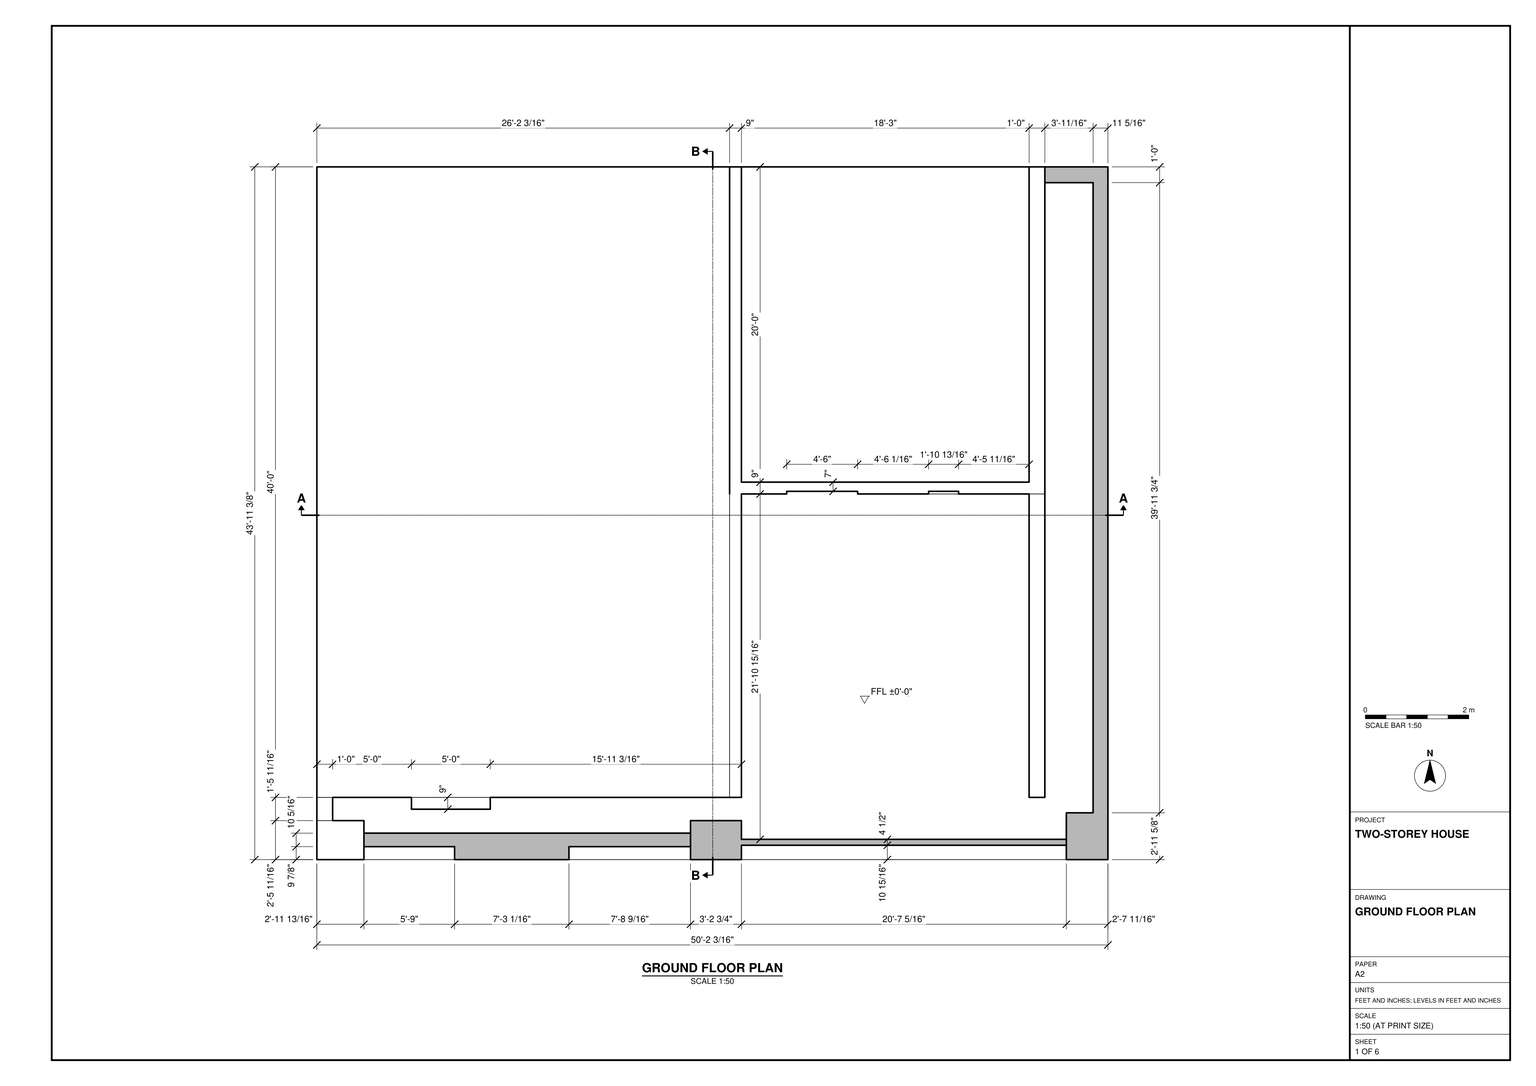
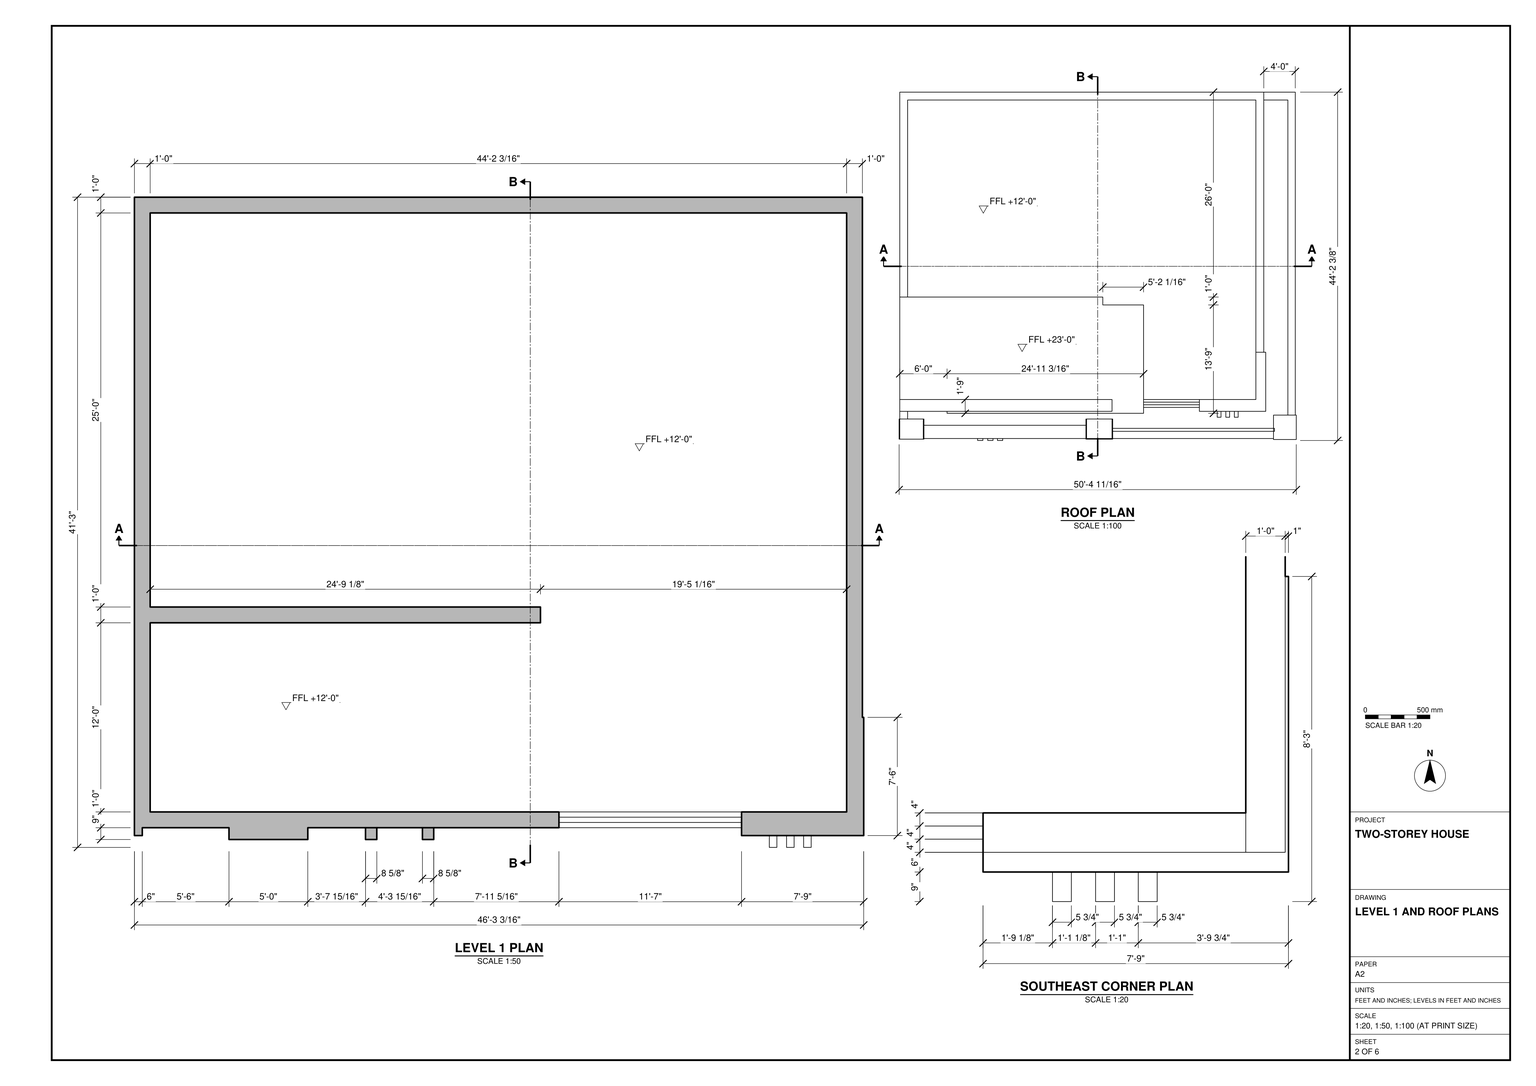
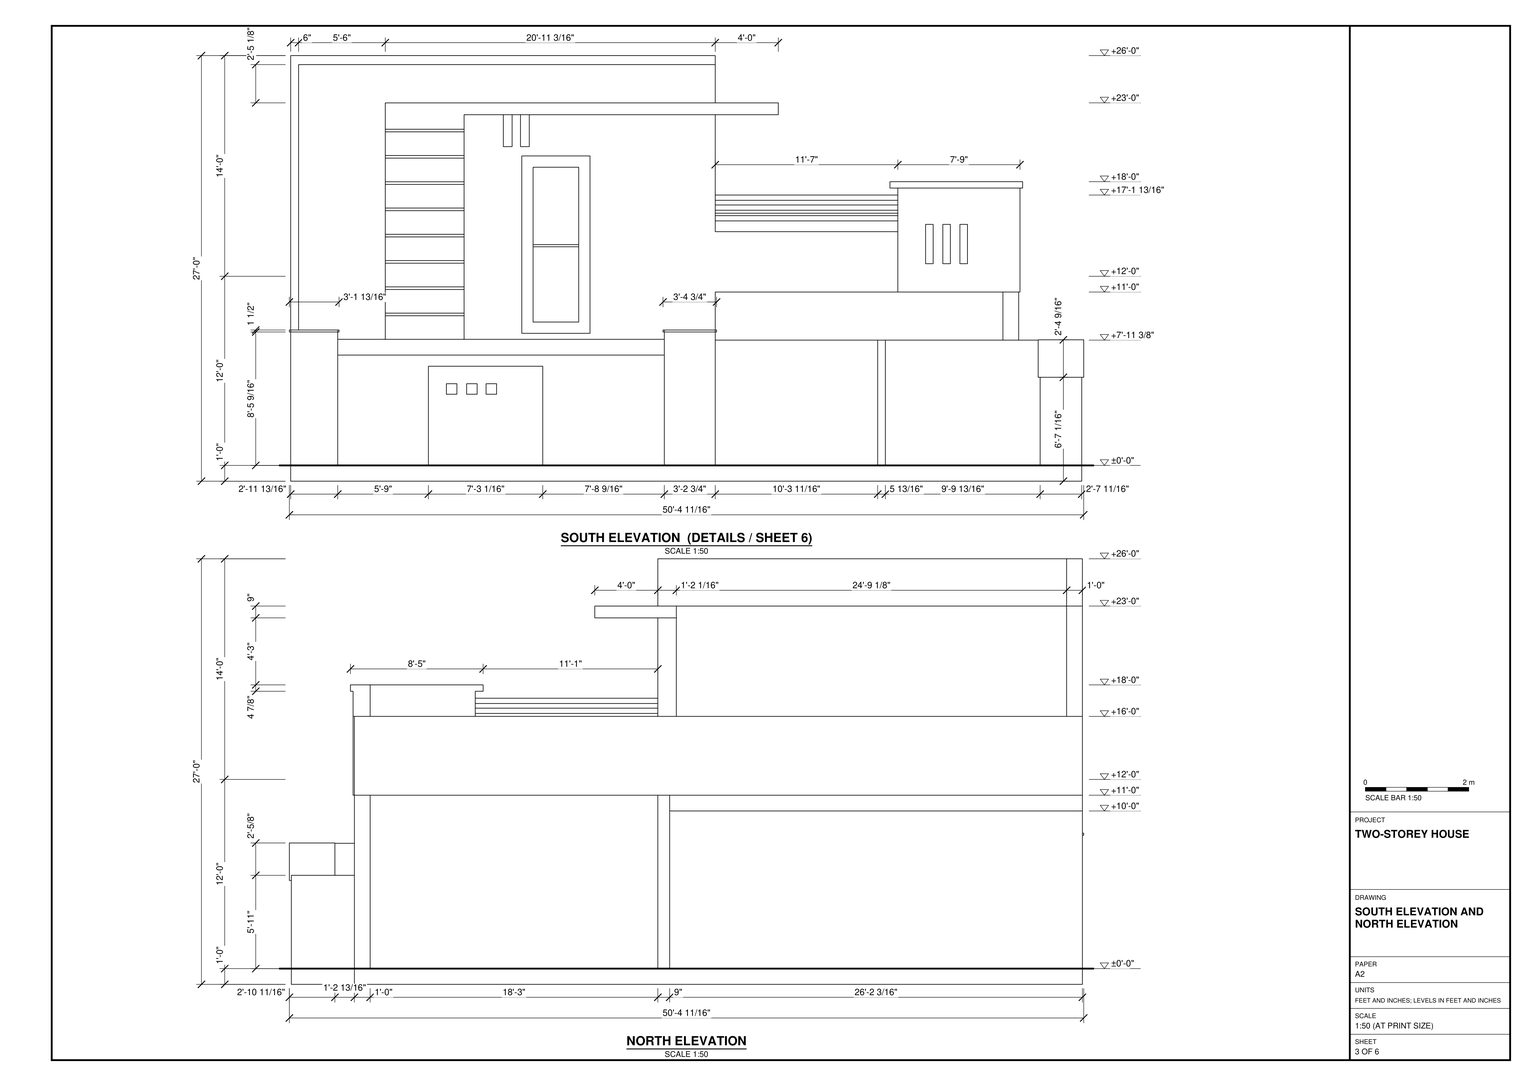
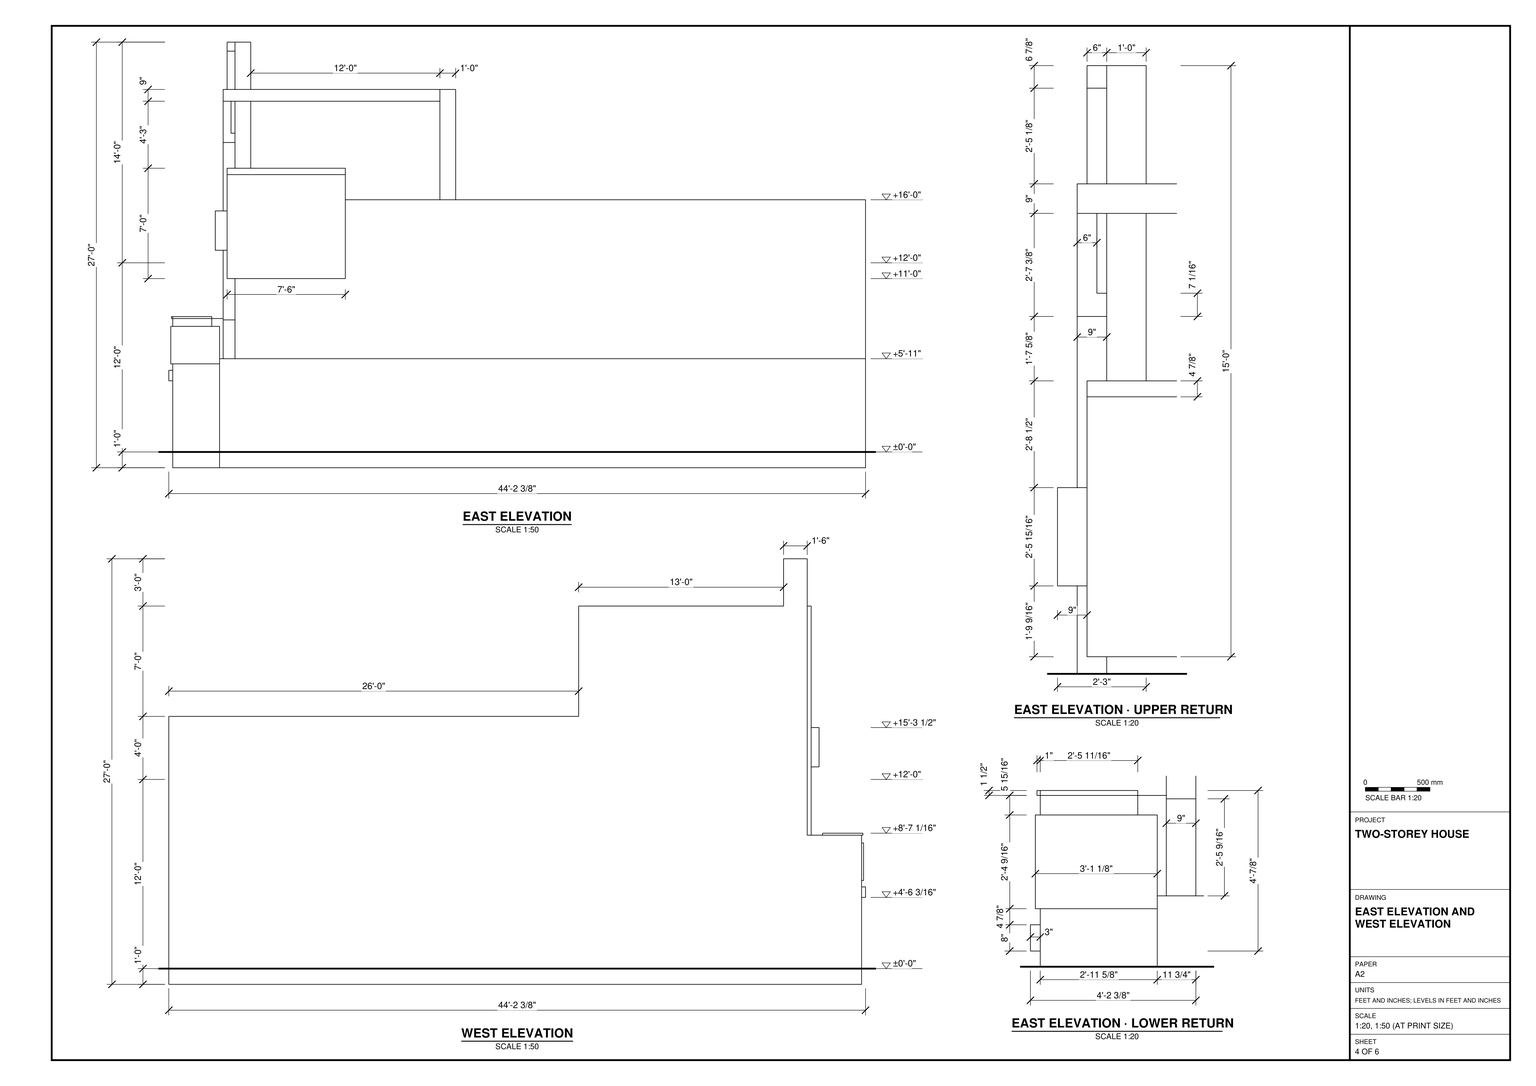
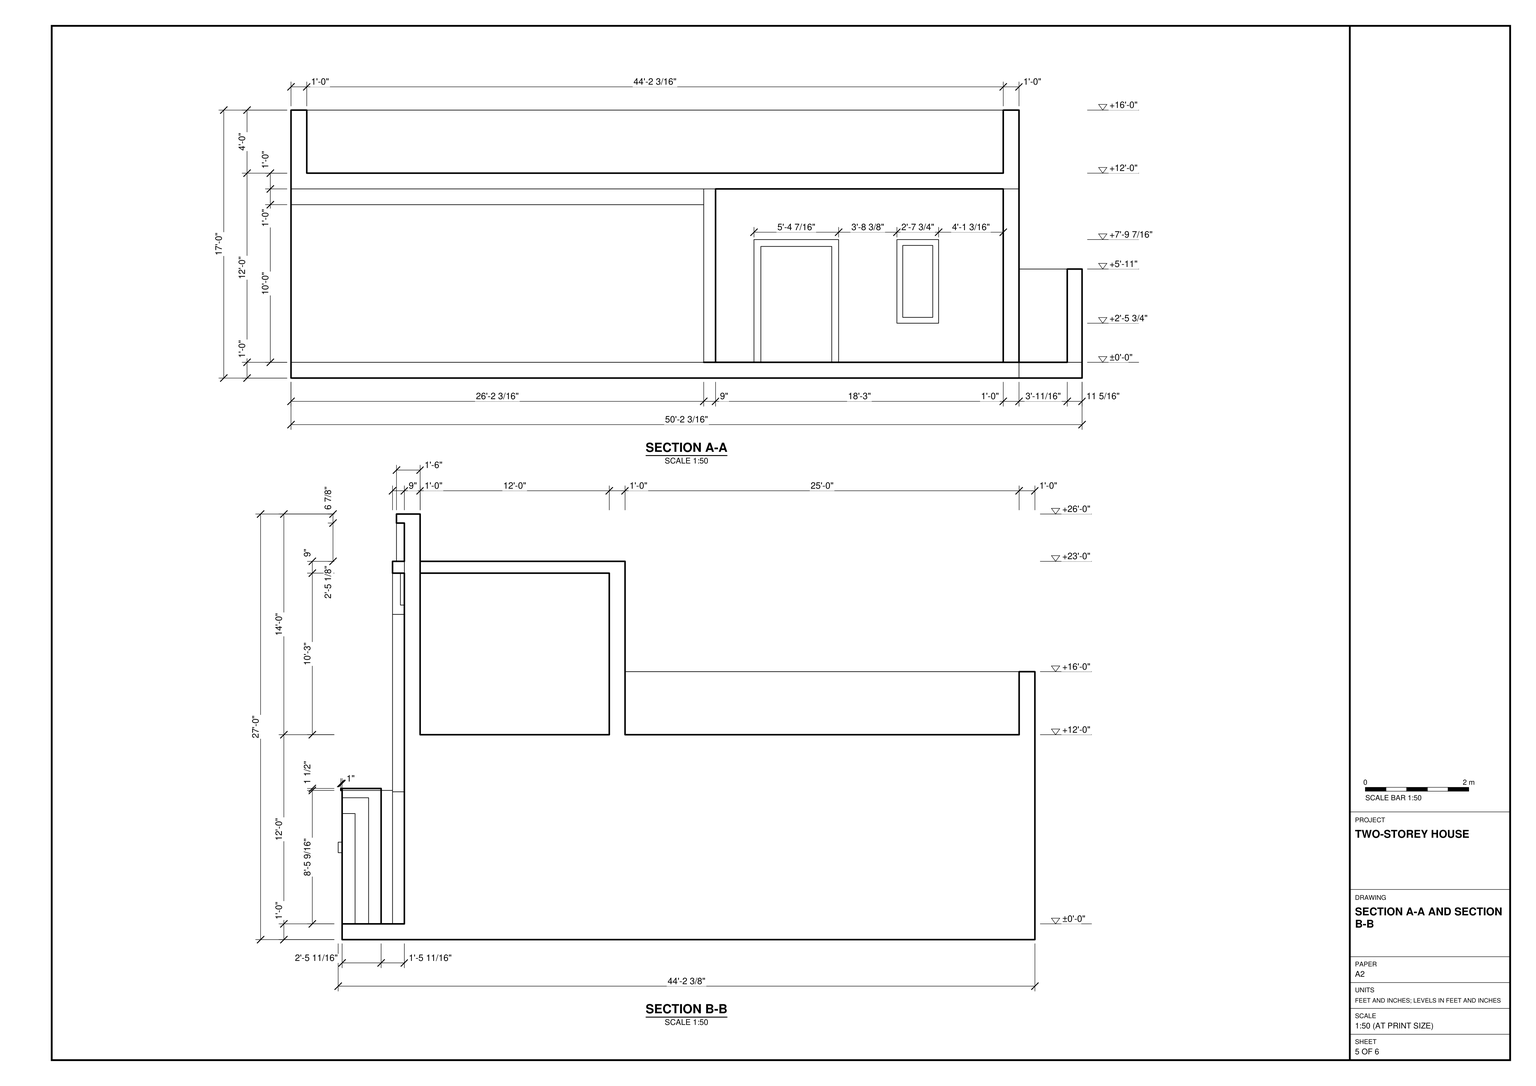
Use task_files/diagram_01.pdf to model the two-storey house in SketchUp. Work in feet and inches. The overall model must measure 50'-4 11/16" east to west, 44'-2 3/8" north to south and 27'-0" from the underside of the base to the highest point. Set the ground-floor finished level at ±0'-0" and the upper floor at +12'-0".

Lay out the broad west bay and the narrower east bay, including the cross wall that divides the east bay. Follow the plans for wall thicknesses, slab edges and openings. Use the roof plan and elevations together to locate the taller front volume, its projecting flat roof and the lower terrace. On the south face, model the horizontal bands beside the tall framed opening. Continue the terrace railing to the solid southeast corner and use the enlarged corner plan to place its narrow vertical details. Model the front boundary wall, piers and gate separately from the house facade, retaining the setbacks shown in plan.

Keep shell elements such as walls, slabs and roof pieces in separate groups or components. Keep each furniture or joinery piece shown separate and use components for repeated parts. Any decor or loose items shown may use suitable library components. Save one SketchUp model as output_files/two_storey_house_with_a_stepped_flat_roof.skp.

# SketchUp Ruby script. Lengths in inches.
U = 1.inch
M = Sketchup.active_model
def pt(a) = Geom::Point3d.new(a.map { |v| v * U })
def face(e, loops, mat)
  f = e.add_face(loops[0].map { |a| pt(a) })
  loops[1..].each { |l| e.add_face(l.map { |a| pt(a) }).erase! }
  f.material = f.back_material = mat if mat
  f
end
# faces: each face lists its corners as indices into pts; further lists are holes
def faces(e, pts, list, mat = nil) = list.each { |f| face(e, (f[0].is_a?(Array) ? f : [f]).map { |l| l.map { |i| pts[i] } }, mat) }
# xy, xz, yz: faces in a plane at the given z, y or x. An outline is a flat list of corners, or four numbers for a rectangle; further outlines are holes
def ring(l) = l.size == 4 ? [[l[0], l[1]], [l[2], l[1]], [l[2], l[3]], [l[0], l[3]]] : l.each_slice(2).to_a
def flat(e, list, mat, &to3) = list.each { |f| face(e, (f[0].is_a?(Array) ? f : [f]).map { |l| ring(l).map { |u, v| to3.(u, v) } }, mat) }
def xy(e, z, list, mat = nil) = flat(e, list, mat) { |x, y| [x, y, z] }
def xz(e, y, list, mat = nil) = flat(e, list, mat) { |x, z| [x, y, z] }
def yz(e, x, list, mat = nil) = flat(e, list, mat) { |y, z| [x, y, z] }
def lines(e, pts, list) = list.each { |a, b| e.add_line(pt(pts[a]), pt(pts[b])) }
# prism: a flat outline (further loops are holes) pulled along v
def prism(e, loops, v, mat = nil)
  f = face(e, loops, mat); d = Geom::Vector3d.new(v.map { |x| x * U })
  f.pushpull(f.normal.samedirection?(d) ? d.length : -d.length)
end
def box(e, o, s, mat = nil) = prism(e, [[o, [o[0] + s[0], o[1], o[2]], [o[0] + s[0], o[1] + s[1], o[2]], [o[0], o[1] + s[1], o[2]]]], [0, 0, s[2]], mat)
def at(x, y, z, deg = 0) = Geom::Transformation.translation(pt([x, y, z])) * Geom::Transformation.rotation(ORIGIN, Z_AXIS, deg.degrees)
def axes(o, x, y, z) = Geom::Transformation.new([*x, 0, *y, 0, *z, 0, *pt(o).to_a, 1])
def part(name) = M.definitions.add(name)
# library, detail: a bought-in or finely detailed component or shape, given as its bounding box
def library(name, o, s) = part(name).tap { |d| box(d.entities, o, s) }
def detail(e, o, s) = box(e.add_group.entities, o, s)
def put(e, d, t, mat = nil) = e.add_instance(d, t).tap { |i| i.material = mat if mat }
def group(e, t, mat = nil) = e.add_group.tap { |g| g.transformation = t; g.material = mat if mat }.entities
root = M.entities
M.materials.add("[0005_LightPink]").color = [255, 182, 193]
M.materials.add("[0008_LavenderBlush]").color = [204, 192, 195]
M.materials.add("[0012_Bisque]").color = [221, 198, 170]
M.materials.add("[0012_Bisque]1").color = [255, 228, 196]
M.materials.add("[0029_BlanchedAlmond]").color = [198, 183, 159]
M.materials.add("[0042_Sienna]").color = [56, 28, 15]
M.materials.add("[0111_SlateGray]").color = [112, 128, 144]
M.materials.add("[0132_LightGray]").color = [169, 169, 169]
M.materials.add("[0134_DimGray]").color = [105, 105, 105]
M.materials.add("[0136_Charcoal]").color = [35, 35, 35]
M.materials.add("[0137_Black]").color = [0, 0, 0]
M.materials.add("[Cladding Siding Tan]").color = [162, 126, 95]
M.materials.add("[Concrete Aggregate Smoke]").color = [154, 150, 148]
M.materials.add("[Stone Flagstone Ashlar]").color = [175, 116, 102]
M.materials.add("[Stone Marble]").color = [143, 138, 136]
M.materials.add("[Translucent Glass Blue]").color = [63, 94, 150]
M.materials["[Translucent Glass Blue]"].alpha = 0.5
M.materials.add("[Translucent Glass Gray]").color = [128, 128, 128]
M.materials["[Translucent Glass Gray]"].alpha = 0.5
xy(root,0,[[1,3,555.1875,50.375],[555.1875,3,603.1875,50.375],[1,50.375,555.1875,530.375],[555.1875,50.375,603.1875,530.375]])
xy(root,12,[[36.8125,3,105.84,12.87],[192.9,3,285.4375,12.87],[285.4375,3,285.4375,32.6875,324.1875,32.6875,324.1875,18.4375,571.53,18.4375,571.53,13.9375,324.1875,13.9375,324.1875,3],[73,41.375,133,50.375],[315.1875,50.375,315.1875,530.375,324.1875,530.375,324.1875,290.375,543.1875,290.375,543.1875,530.375,555.1875,530.375,555.1875,281.375,412.64,281.375,412.64,283.375,358.66,283.375,358.66,281.375,324.1875,281.375,324.1875,50.375],
  [543.1875,50.375,555.1875,281.375],[324.1875,290.375,543.1875,530.375]])
xy(root,12,[[324.1875,3,571.53,13.9375]],"[0111_SlateGray]")
xy(root,12,[[324.1875,18.4375,571.53,18.4375,571.53,38.625,591.9,38.625,591.9,518.375,555.1875,518.375,555.1875,50.375,543.1875,50.375,543.1875,281.375,412.64,281.375,412.64,283.375,358.66,283.375,358.66,281.375,324.1875,281.375,324.1875,50.375,133,50.375,133,41.375,73,41.375,73,50.375,13,50.375,13,32.6875,36.8125,32.6875,36.8125,23.15,285.4375,23.15,285.4375,32.6875,324.1875,32.6875]],"[Stone Marble]")
xy(root,46.21,[[466.69,281.375,489.53,283.375]],"[0029_BlanchedAlmond]")
xy(root,66.19,[[119.53,0,127.53,3],[134.93,0,142.93,3],[149.74,0,157.74,3]])
xy(root,74.19,[[119.53,0,127.53,3],[134.93,0,142.93,3],[149.74,0,157.74,3]])
xy(root,79.08,[[570.03,3,571.53,38.625]])
xy(root,79.08,[[570.03,1.5,604.6875,3],[603.1875,3,604.6875,38.625]],"[0012_Bisque]")
xy(root,83,[[591.9,38.625,603.1875,38.625,603.1875,530.375,555.1875,530.375,555.1875,518.375,591.9,518.375]])
xy(root,87.5,[[105.84,3,192.9,12.87]])
xy(root,96,[[36.8125,3,285.4375,12.87]])
xy(root,100.21,[[358.66,281.375,412.64,283.375]],"[0042_Sienna]")
xy(root,100.98,[[466.69,281.375,489.53,283.375]])
xy(root,107.375,[[324.1875,13.9375,571.53,18.4375]],"[0136_Charcoal]")
xy(root,107.625,[[570.03,1.5,604.6875,38.625]],"[0012_Bisque]")
xy(root,108,[[36.8125,3,285.4375,23.15]],"[0029_BlanchedAlmond]")
xy(root,112.55,[[176.93,41.375,228.86,50.375]],"[0132_LightGray]")
xy(root,113.58,[[284.4375,2,285.4375,3],[284.4375,3,285.4375,32.6875],[1,32.6875,13,32.6875,13,50.375,7,50.375,7,44.375,1,44.375]])
xy(root,113.58,[[0,2,1,3],[1,2,36.8125,3],[36.8125,2,37.8125,3],[285.4375,2,324.1875,3],[324.1875,2,325.1875,3],
  [0,3,1,32.6875],[36.8125,3,37.8125,32.6875],[324.1875,3,325.1875,32.6875]],"[0029_BlanchedAlmond]")
xy(root,115.08,[[0,2,1,32.6875]])
xy(root,115.08,[[1,2,36.8125,32.6875],[36.8125,2,37.8125,32.6875],[284.4375,2,285.4375,3],[285.4375,2,324.1875,3],[324.1875,2,325.1875,3],
  [284.4375,3,285.4375,32.6875],[285.4375,3,324.1875,32.6875],[324.1875,3,325.1875,32.6875]],"[0029_BlanchedAlmond]")
xy(root,121.15,[[185.52,41.375,220.26,50.375]],"[0042_Sienna]")
xy(root,144,[[324.1875,290.375,543.1875,530.375]])
xy(root,144,[[[324.1875,50.375,543.1875,281.375],[360.1875,86.375,507.1875,245.375]]],"[0005_LightPink]")
xy(root,144,[[463.1875,44.375,463.1875,50.375,555.1875,50.375,555.1875,134.375,556.1875,134.375,556.1875,44.375]],"[0042_Sienna]")
xy(root,150,[[[360.1875,86.375,507.1875,245.375],[386.07,209.3125,387.58,209.7,388.95,210.47,390.0625,211.57,390.86,212.92,391.28,214.43,391.3,215.99,390.9,217.51,390.13,218.875,389.04,219.99,387.6875,220.79,386.18,221.21,384.61,221.22,383.1,220.83,381.73,220.0625,380.61,218.97,379.82,217.62,379.4,216.11,379.38,214.54,379.77,213.02,380.54,211.66,381.64,210.54,382.99,209.75,384.5,209.33],[489.19,109.125,490.71,109.52,492.07,110.29,493.1875,111.38,493.99,112.73,494.41,114.24,494.42,115.81,494.03,117.32,493.26,118.6875,492.16,119.81,490.8125,120.6,489.3,121.02,487.74,121.04,486.22,120.65,484.86,119.875,483.74,118.78,482.94,117.43,482.52,115.92,482.51,114.35,482.9,112.84,483.67,111.47,484.77,110.36,486.12,109.56,487.625,109.14],[391.5,109.125,393.02,109.52,394.38,110.29,395.5,111.38,396.3,112.73,396.72,114.24,396.73,115.81,396.34,117.32,395.57,118.6875,394.47,119.81,393.125,120.6,391.62,121.02,390.05,121.04,388.53,120.65,387.17,119.875,386.05,118.78,385.26,117.43,384.84,115.92,384.82,114.35,385.21,112.84,385.98,111.47,387.08,110.36,388.43,109.56,389.9375,109.14],[489.19,209.3125,490.71,209.7,492.07,210.47,493.1875,211.57,493.99,212.92,494.41,214.43,494.42,215.99,494.03,217.51,493.26,218.875,492.16,219.99,490.8125,220.79,489.3,221.21,487.74,221.22,486.22,220.83,484.86,220.0625,483.74,218.97,482.94,217.62,482.52,216.11,482.51,214.54,482.9,213.02,483.67,211.66,484.77,210.54,486.12,209.75,487.625,209.33]]],"[0008_LavenderBlush]")
xy(root,151,[[391.5,109.125,389.9375,109.14,388.43,109.56,387.08,110.36,385.98,111.47,385.21,112.84,384.82,114.35,384.84,115.92,385.26,117.43,386.05,118.78,387.17,119.875,388.53,120.65,390.05,121.04,391.62,121.02,393.125,120.6,394.47,119.81,395.57,118.6875,396.34,117.32,396.73,115.81,396.72,114.24,396.3,112.73,395.5,111.38,394.38,110.29,393.02,109.52],[489.19,109.125,487.625,109.14,486.12,109.56,484.77,110.36,483.67,111.47,482.9,112.84,482.51,114.35,482.52,115.92,482.94,117.43,483.74,118.78,484.86,119.875,486.22,120.65,487.74,121.04,489.3,121.02,490.8125,120.6,492.16,119.81,493.26,118.6875,494.03,117.32,494.42,115.81,494.41,114.24,493.99,112.73,493.1875,111.38,492.07,110.29,490.71,109.52],[386.07,209.3125,384.5,209.33,382.99,209.75,381.64,210.54,380.54,211.66,379.77,213.02,379.38,214.54,379.4,216.11,379.82,217.62,380.61,218.97,381.73,220.0625,383.1,220.83,384.61,221.22,386.18,221.21,387.6875,220.79,389.04,219.99,390.13,218.875,390.9,217.51,391.3,215.99,391.28,214.43,390.86,212.92,390.0625,211.57,388.95,210.47,387.58,209.7],[489.19,209.3125,487.625,209.33,486.12,209.75,484.77,210.54,483.67,211.66,482.9,213.02,482.51,214.54,482.52,216.11,482.94,217.62,483.74,218.97,484.86,220.0625,486.22,220.83,487.74,221.22,489.3,221.21,490.8125,220.79,492.16,219.99,493.26,218.875,494.03,217.51,494.42,215.99,494.41,214.43,493.99,212.92,493.1875,211.57,492.07,210.47,490.71,209.7]])
xy(root,156,[[13,62.375,543.1875,62.375,543.1875,518.375,13,518.375,13,218.375,310.11,218.375,310.11,206.375,13,206.375]])
xy(root,165.5625,[[484.33,35.375,490.08,44.375],[497.45,35.375,503.2,44.375],[510.45,35.375,516.2,44.375]])
xy(root,189.9375,[[324.1875,50.375,463.1875,62.375]],"[0012_Bisque]1")
xy(root,195.5,[[484.33,35.375,490.08,44.375],[497.45,35.375,503.2,44.375],[510.45,35.375,516.2,44.375]])
xy(root,204,[[543.1875,134.375,555.1875,134.375,555.1875,530.375,1,530.375,1,218.375,13,218.375,13,518.375,543.1875,518.375]])
xy(root,223.15,[[457.1875,44.375,463.1875,62.375]])
xy(root,223.15,[[556.1875,44.375,558.1875,134.375]],"[0042_Sienna]")
xy(root,228,[[457.1875,44.375,558.1875,44.375,558.1875,134.375,543.1875,134.375,543.1875,62.375,457.1875,62.375]],"[0012_Bisque]1")
xy(root,239.01,[[185.52,41.375,220.26,50.375]],"[0042_Sienna]")
xy(root,247.61,[[176.93,41.375,228.86,50.375]],"[0132_LightGray]")
xy(root,254.6875,[[162.875,47.375,169.5625,50.375],[175.9375,47.375,182.625,50.375]])
xy(root,279,[[347.08,69.3,345.51,69.37,344.02,69.84,342.7,70.68,341.64,71.84,340.92,73.23,340.58,74.76,340.65,76.32,341.12,77.82,341.96,79.14,343.12,80.2,344.51,80.92,346.04,81.26,347.6,81.1875,349.1,80.71,350.42,79.87,351.47,78.72,352.2,77.33,352.53,75.8,352.47,74.23,351.99,72.74,351.15,71.42,350,70.36,348.61,69.64],[347.08,142.43,345.51,142.49,344.02,142.97,342.7,143.81,341.64,144.96,340.92,146.35,340.58,147.88,340.65,149.45,341.12,150.94,341.96,152.26,343.12,153.32,344.51,154.04,346.04,154.38,347.6,154.3125,349.1,153.84,350.42,153,351.47,151.84,352.2,150.45,352.53,148.92,352.47,147.36,351.99,145.86,351.15,144.54,350,143.49,348.61,142.76]])
xy(root,279,[[[133,41.375,133,50.375,162.875,50.375,162.875,47.375,169.5625,47.375,169.5625,50.375,175.9375,50.375,175.9375,47.375,182.625,47.375,182.625,50.375,324.1875,50.375,324.1875,62.375,13,62.375,13,206.375,372.1875,206.375,372.1875,41.375],[347.08,69.3,348.61,69.64,350,70.36,351.15,71.42,351.99,72.74,352.47,74.23,352.53,75.8,352.2,77.33,351.47,78.72,350.42,79.87,349.1,80.71,347.6,81.1875,346.04,81.26,344.51,80.92,343.12,80.2,341.96,79.14,341.12,77.82,340.65,76.32,340.58,74.76,340.92,73.23,341.64,71.84,342.7,70.68,344.02,69.84,345.51,69.37],[347.08,142.43,348.61,142.76,350,143.49,351.15,144.54,351.99,145.86,352.47,147.36,352.53,148.92,352.2,150.45,351.47,151.84,350.42,153,349.1,153.84,347.6,154.3125,346.04,154.38,344.51,154.04,343.12,153.32,341.96,152.26,341.12,150.94,340.65,149.45,340.58,147.88,340.92,146.35,341.64,144.96,342.7,143.81,344.02,142.97,345.51,142.49]]],"[0042_Sienna]")
xy(root,288,[[73,41.375,372.1875,41.375,372.1875,206.375,310.11,206.375,310.11,218.375,1,218.375,1,62.375,324.1875,62.375,324.1875,50.375,73,50.375]],"[0012_Bisque]1")
xy(root,317.13,[[7,44.375,324.1875,50.375]],"[0134_DimGray]")
xy(root,324,[[1,44.375,324.1875,62.375]],"[0012_Bisque]1")
xz(root,0,[[119.53,66.19,127.53,74.19],[134.93,66.19,142.93,74.19],[149.74,66.19,157.74,74.19]])
xz(root,1.5,[[570.03,79.08,604.6875,107.625]],"[0012_Bisque]")
xz(root,2,[[0,113.58,1,115.08],[1,113.58,36.8125,115.08],[36.8125,113.58,37.8125,115.08],[284.4375,113.58,285.4375,115.08],[285.4375,113.58,324.1875,115.08],
  [324.1875,113.58,325.1875,115.08]],"[0029_BlanchedAlmond]")
xz(root,3,[[[105.84,12,192.9,87.5],[119.53,66.19,127.53,74.19],[134.93,66.19,142.93,74.19],[149.74,66.19,157.74,74.19]],[284.4375,113.58,285.4375,115.08],[285.4375,113.58,324.1875,115.08],[324.1875,113.58,325.1875,115.08]])
xz(root,3,[[36.8125,96,285.4375,108]],"[0029_BlanchedAlmond]")
xz(root,3,[[1,0,603.1875,0,603.1875,79.08,571.53,79.08,571.53,12,36.8125,12,36.8125,113.58,1,113.58],[285.4375,12,324.1875,113.58]],"[Stone Flagstone Ashlar]")
xz(root,12.87,[[36.8125,12,105.84,12,105.84,87.5,192.9,87.5,192.9,12,285.4375,12,285.4375,96,36.8125,96]],"[Concrete Aggregate Smoke]")
xz(root,13.9375,[[447.86,12,453.7,107.375]],"[0136_Charcoal]")
xz(root,13.9375,[[324.1875,12,447.86,107.375],[453.7,12,571.53,107.375]],"[Cladding Siding Tan]")
xz(root,18.4375,[[324.1875,12,571.53,107.375]])
xz(root,23.15,[[36.8125,12,285.4375,108]])
xz(root,32.6875,[[13,12,13,113.58,1,113.58,1,115.08,36.8125,115.08,36.8125,12],[285.4375,12,324.1875,115.08],[0,113.58,1,115.08],[36.8125,113.58,37.8125,115.08],[284.4375,113.58,285.4375,115.08],
  [324.1875,113.58,325.1875,115.08]])
xz(root,35.375,[[484.33,165.5625,490.08,195.5],[497.45,165.5625,503.2,195.5],[510.45,165.5625,516.2,195.5]])
xz(root,38.625,[[571.53,12,571.53,79.08,570.03,79.08,570.03,83,591.9,83,591.9,12],[603.1875,79.08,603.1875,83,570.03,83,570.03,107.625,604.6875,107.625,604.6875,79.08]])
xz(root,41.375,[[73,125.9375,133,127.9375],[73,145.9375,133,147.9375],[73,165.9375,133,167.9375],[73,185.9375,133,187.9375],[73,205.9375,133,207.9375],
  [73,225.9375,133,227.9375],[73,245.9375,133,247.9375],[73,265.9375,133,267.9375]])
xz(root,41.375,[[73,12,133,125.9375],[73,127.9375,133,145.9375],[73,147.9375,133,165.9375],[73,167.9375,133,185.9375],[73,187.9375,133,205.9375],
  [73,207.9375,133,225.9375],[73,227.9375,133,245.9375],[73,247.9375,133,265.9375],[73,267.9375,133,267.9375,133,279,372.1875,279,372.1875,288,73,288]],"[0042_Sienna]")
xz(root,41.375,[[[176.93,112.55,228.86,247.61],[185.52,121.15,220.26,239.01]]],"[0132_LightGray]")
xz(root,44.375,[[484.33,165.5625,490.08,195.5],[497.45,165.5625,503.2,195.5],[510.45,165.5625,516.2,195.5]])
xz(root,44.375,[[[463.1875,144,556.1875,223.15],[484.33,165.5625,490.08,195.5],[497.45,165.5625,503.2,195.5],[510.45,165.5625,516.2,195.5]],[457.1875,223.15,558.1875,228]],"[0042_Sienna]")
xz(root,44.375,[[1,113.58,7,113.58,7,317.13,324.1875,317.13,324.1875,324,1,324]],"[0134_DimGray]")
xz(root,47.375,[[162.875,254.6875,169.5625,279],[175.9375,254.6875,182.625,279]])
xz(root,50.375,[[[176.93,112.55,228.86,247.61],[185.52,121.15,220.26,239.01]],[185.52,178.46,220.26,180.08]])
xz(root,50.375,[[13,12,73,12,73,288,324.1875,288,324.1875,317.13,7,317.13,7,113.58,13,113.58],[[133,12,324.1875,12,324.1875,144,463.1875,144,463.1875,189.9375,324.1875,189.9375,324.1875,279,182.625,279,182.625,254.6875,175.9375,254.6875,175.9375,279,169.5625,279,169.5625,254.6875,162.875,254.6875,162.875,279,133,279],[176.93,112.55,228.86,247.61]],[543.1875,12,555.1875,144]],"[0029_BlanchedAlmond]")
xz(root,50.375,[[185.52,121.15,220.26,178.46],[185.52,180.08,220.26,239.01]],"[Translucent Glass Blue]")
xz(root,62.375,[[324.1875,156,324.1875,189.9375,463.1875,189.9375,463.1875,204,543.1875,204,543.1875,156],[463.1875,204,463.1875,223.15,457.1875,223.15,457.1875,228,543.1875,228,543.1875,204],[13,279,324.1875,288],[1,288,13,324]])
xz(root,62.375,[[13,156,324.1875,279],[13,288,324.1875,324]],"[0012_Bisque]1")
xz(root,86.375,[[360.1875,144,507.1875,150]])
xz(root,134.375,[[555.1875,144,556.1875,204],[543.1875,204,543.1875,228,558.1875,228,558.1875,223.15,556.1875,223.15,556.1875,204]])
xz(root,206.375,[[310.11,279,372.1875,288]])
xz(root,206.375,[[13,156,310.11,279]],"[0012_Bisque]1")
xz(root,218.375,[[13,156,310.11,288],[1,204,13,288]])
xz(root,245.375,[[360.1875,144,507.1875,150]],"[0008_LavenderBlush]")
xz(root,281.375,[[[324.1875,12,353.43,12,353.43,105.4375,417.87,105.4375,417.87,12,543.1875,12,543.1875,144,324.1875,144],[462.23,41.75,493.98,105.4375]],[[462.23,41.75,493.98,105.4375],[466.69,46.21,489.53,100.98]]],"[0029_BlanchedAlmond]")
xz(root,281.375,[[353.43,12,358.66,12,358.66,100.21,412.64,100.21,412.64,12,417.87,12,417.87,105.4375,353.43,105.4375]],"[0042_Sienna]")
xz(root,283.375,[[358.66,12,412.64,100.21]],"[0042_Sienna]")
xz(root,283.375,[[466.69,46.21,489.53,100.98]],"[Translucent Glass Gray]")
xz(root,290.375,[[324.1875,12,543.1875,144]])
xz(root,518.375,[[13,156,543.1875,204]])
xz(root,518.375,[[555.1875,12,591.9,83]],"[0029_BlanchedAlmond]")
xz(root,530.375,[[1,0,555.1875,12],[555.1875,0,603.1875,12],[1,12,315.1875,132],[315.1875,12,324.1875,144],[324.1875,12,543.1875,144],
  [543.1875,12,555.1875,144],[555.1875,12,603.1875,83],[1,132,315.1875,144],[1,144,555.1875,204]])
yz(root,0,[[2,113.58,32.6875,115.08]],"[0029_BlanchedAlmond]")
yz(root,1,[[3,0,3,113.58,44.375,113.58,44.375,324,62.375,324,62.375,288,218.375,288,218.375,204,530.375,204,530.375,0],[2,113.58,32.6875,115.08]])
yz(root,7,[[44.375,113.58,50.375,317.13]],"[0134_DimGray]")
yz(root,13,[[32.6875,12,50.375,113.58],[62.375,156,206.375,279],[218.375,156,518.375,204]])
yz(root,36.8125,[[12.87,12,23.15,12,23.15,108,3,108,3,96,12.87,96],[2,113.58,32.6875,115.08]])
yz(root,36.8125,[[23.15,12,32.6875,12,32.6875,113.58,3,113.58,3,108,23.15,108]],"[0111_SlateGray]")
yz(root,36.8125,[[3,12,12.87,96]],"[Stone Flagstone Ashlar]")
yz(root,37.8125,[[2,113.58,32.6875,115.08]],"[0029_BlanchedAlmond]")
yz(root,73,[[41.375,12,50.375,288]],"[0042_Sienna]")
yz(root,105.84,[[3,12,12.87,87.5]])
yz(root,119.53,[[0,66.19,3,74.19]])
yz(root,127.53,[[0,66.19,3,74.19]])
yz(root,133,[[41.375,12,50.375,279]],"[0042_Sienna]")
yz(root,134.93,[[0,66.19,3,74.19]])
yz(root,142.93,[[0,66.19,3,74.19]])
yz(root,149.74,[[0,66.19,3,74.19]])
yz(root,157.74,[[0,66.19,3,74.19]])
yz(root,162.875,[[47.375,254.6875,50.375,279]])
yz(root,169.5625,[[47.375,254.6875,50.375,279]])
yz(root,175.9375,[[47.375,254.6875,50.375,279]])
yz(root,176.93,[[41.375,112.55,50.375,247.61]],"[0132_LightGray]")
yz(root,182.625,[[47.375,254.6875,50.375,279]])
yz(root,185.52,[[41.375,121.15,50.375,239.01]],"[0042_Sienna]")
yz(root,192.9,[[3,12,12.87,87.5]])
yz(root,220.26,[[41.375,121.15,50.375,239.01]],"[0042_Sienna]")
yz(root,228.86,[[41.375,112.55,50.375,247.61]],"[0132_LightGray]")
yz(root,284.4375,[[2,113.58,3,115.08],[3,113.58,32.6875,115.08]],"[0029_BlanchedAlmond]")
yz(root,285.4375,[[12.87,12,12.87,96,3,96,3,108,23.15,108,23.15,12],[23.15,12,23.15,108,3,108,3,113.58,32.6875,113.58,32.6875,12],[2,113.58,3,115.08],[3,113.58,32.6875,115.08]])
yz(root,285.4375,[[3,12,12.87,96]],"[Stone Flagstone Ashlar]")
yz(root,310.11,[[206.375,156,218.375,288]],"[0012_Bisque]1")
yz(root,315.1875,[[281.375,12,530.375,132],[281.375,132,530.375,144]])
yz(root,324.1875,[[290.375,12,530.375,144],[2,113.58,3,115.08],[3,113.58,32.6875,115.08],[50.375,279,62.375,288]])
yz(root,324.1875,[[[50.375,189.9375,62.375,279],[56.375,198.15,55.86,198.21,55.375,198.41,54.96,198.73,54.64,199.15,54.44,199.63,54.375,200.15,54.44,200.66,54.64,201.15,54.96,201.56,55.375,201.88,55.86,202.08,56.375,202.15,56.89,202.08,57.375,201.88,57.79,201.56,58.11,201.15,58.31,200.66,58.375,200.15,58.31,199.63,58.11,199.15,57.79,198.73,57.375,198.41,56.89,198.21],[56.375,206.27,55.86,206.34,55.375,206.54,54.96,206.86,54.64,207.27,54.44,207.75,54.375,208.27,54.44,208.79,54.64,209.27,54.96,209.68,55.375,210,55.86,210.2,56.375,210.27,56.89,210.2,57.375,210,57.79,209.68,58.11,209.27,58.31,208.79,58.375,208.27,58.31,207.75,58.11,207.27,57.79,206.86,57.375,206.54,56.89,206.34],[56.375,213.83,55.86,213.9,55.375,214.1,54.96,214.42,54.64,214.83,54.44,215.32,54.375,215.83,54.44,216.35,54.64,216.83,54.96,217.25,55.375,217.56,55.86,217.76,56.375,217.83,56.89,217.76,57.375,217.56,57.79,217.25,58.11,216.83,58.31,216.35,58.375,215.83,58.31,215.32,58.11,214.83,57.79,214.42,57.375,214.1,56.89,213.9]],[50.375,288,62.375,324],[44.375,317.13,50.375,324]],"[0012_Bisque]1")
yz(root,324.1875,[[50.375,12,281.375,144]],"[0029_BlanchedAlmond]")
yz(root,324.1875,[[3,12,13.9375,12,13.9375,107.375,18.4375,107.375,18.4375,12,32.6875,12,32.6875,113.58,3,113.58]],"[Stone Flagstone Ashlar]")
yz(root,325.1875,[[2,113.58,3,115.08],[3,113.58,32.6875,115.08]],"[0029_BlanchedAlmond]")
yz(root,358.66,[[281.375,12,283.375,100.21]],"[0042_Sienna]")
yz(root,360.1875,[[86.375,144,245.375,150]],"[0008_LavenderBlush]")
yz(root,372.1875,[[41.375,279,206.375,288]],"[0012_Bisque]1")
yz(root,412.64,[[281.375,12,283.375,100.21]],"[0042_Sienna]")
yz(root,457.1875,[[44.375,223.15,62.375,228]],"[0042_Sienna]")
yz(root,463.1875,[[56.375,198.15,56.89,198.21,57.375,198.41,57.79,198.73,58.11,199.15,58.31,199.63,58.375,200.15,58.31,200.66,58.11,201.15,57.79,201.56,57.375,201.88,56.89,202.08,56.375,202.15,55.86,202.08,55.375,201.88,54.96,201.56,54.64,201.15,54.44,200.66,54.375,200.15,54.44,199.63,54.64,199.15,54.96,198.73,55.375,198.41,55.86,198.21],[56.375,206.27,56.89,206.34,57.375,206.54,57.79,206.86,58.11,207.27,58.31,207.75,58.375,208.27,58.31,208.79,58.11,209.27,57.79,209.68,57.375,210,56.89,210.2,56.375,210.27,55.86,210.2,55.375,210,54.96,209.68,54.64,209.27,54.44,208.79,54.375,208.27,54.44,207.75,54.64,207.27,54.96,206.86,55.375,206.54,55.86,206.34],[56.375,213.83,56.89,213.9,57.375,214.1,57.79,214.42,58.11,214.83,58.31,215.32,58.375,215.83,58.31,216.35,58.11,216.83,57.79,217.25,57.375,217.56,56.89,217.76,56.375,217.83,55.86,217.76,55.375,217.56,54.96,217.25,54.64,216.83,54.44,216.35,54.375,215.83,54.44,215.32,54.64,214.83,54.96,214.42,55.375,214.1,55.86,213.9]])
yz(root,463.1875,[[[44.375,144,44.375,223.15,62.375,223.15,62.375,189.9375,50.375,189.9375,50.375,144],[56.375,206.27,56.89,206.34,57.375,206.54,57.79,206.86,58.11,207.27,58.31,207.75,58.375,208.27,58.31,208.79,58.11,209.27,57.79,209.68,57.375,210,56.89,210.2,56.375,210.27,55.86,210.2,55.375,210,54.96,209.68,54.64,209.27,54.44,208.79,54.375,208.27,54.44,207.75,54.64,207.27,54.96,206.86,55.375,206.54,55.86,206.34],[56.375,213.83,56.89,213.9,57.375,214.1,57.79,214.42,58.11,214.83,58.31,215.32,58.375,215.83,58.31,216.35,58.11,216.83,57.79,217.25,57.375,217.56,56.89,217.76,56.375,217.83,55.86,217.76,55.375,217.56,54.96,217.25,54.64,216.83,54.44,216.35,54.375,215.83,54.44,215.32,54.64,214.83,54.96,214.42,55.375,214.1,55.86,213.9],[56.375,198.15,56.89,198.21,57.375,198.41,57.79,198.73,58.11,199.15,58.31,199.63,58.375,200.15,58.31,200.66,58.11,201.15,57.79,201.56,57.375,201.88,56.89,202.08,56.375,202.15,55.86,202.08,55.375,201.88,54.96,201.56,54.64,201.15,54.44,200.66,54.375,200.15,54.44,199.63,54.64,199.15,54.96,198.73,55.375,198.41,55.86,198.21]]],"[0042_Sienna]")
yz(root,466.69,[[281.375,46.21,283.375,100.98]],"[0029_BlanchedAlmond]")
yz(root,484.33,[[35.375,165.5625,44.375,195.5]])
yz(root,489.53,[[281.375,46.21,283.375,100.98]],"[0029_BlanchedAlmond]")
yz(root,490.08,[[35.375,165.5625,44.375,195.5]])
yz(root,497.45,[[35.375,165.5625,44.375,195.5]])
yz(root,503.2,[[35.375,165.5625,44.375,195.5]])
yz(root,507.1875,[[86.375,144,245.375,150]],"[0008_LavenderBlush]")
yz(root,510.45,[[35.375,165.5625,44.375,195.5]])
yz(root,516.2,[[35.375,165.5625,44.375,195.5]])
yz(root,543.1875,[[290.375,12,530.375,144],[62.375,156,518.375,204],[62.375,204,134.375,228]])
yz(root,543.1875,[[50.375,12,281.375,144]],"[0029_BlanchedAlmond]")
yz(root,555.1875,[[518.375,12,530.375,83]])
yz(root,555.1875,[[50.375,12,518.375,12,518.375,83,530.375,83,530.375,204,134.375,204,134.375,144,50.375,144]],"[0029_BlanchedAlmond]")
yz(root,556.1875,[[44.375,144,134.375,223.15]],"[0042_Sienna]")
yz(root,558.1875,[[44.375,223.15,134.375,228]],"[0042_Sienna]")
yz(root,570.03,[[1.5,79.08,13.9375,107.625],[13.9375,79.08,38.625,107.625]],"[0012_Bisque]")
yz(root,571.53,[[13.9375,12,18.4375,79.08],[18.4375,12,38.625,79.08],[13.9375,79.08,18.4375,107.375]])
yz(root,571.53,[[3,12,13.9375,79.08]],"[Stone Flagstone Ashlar]")
yz(root,591.9,[[38.625,12,518.375,83]],"[0029_BlanchedAlmond]")
yz(root,603.1875,[[3,0,38.625,79.08],[38.625,0,530.375,83]])
yz(root,604.6875,[[1.5,79.08,38.625,107.625]],"[0012_Bisque]")
p = [[389.9375,109.14,150],[388.43,109.56,150],[388.43,109.56,151],[389.9375,109.14,151],[391.5,109.125,150],[391.5,109.125,151],
  [393.02,109.52,150],[393.02,109.52,151],[487.625,109.14,150],[486.12,109.56,150],[486.12,109.56,151],[487.625,109.14,151],
  [489.19,109.125,150],[489.19,109.125,151],[490.71,109.52,150],[490.71,109.52,151],[394.38,110.29,150],[394.38,110.29,151],
  [492.07,110.29,150],[492.07,110.29,151],[387.08,110.36,150],[387.08,110.36,151],[484.77,110.36,150],[484.77,110.36,151],
  [395.5,111.38,150],[395.5,111.38,151],[493.1875,111.38,150],[493.1875,111.38,151],[385.98,111.47,150],[385.98,111.47,151],
  [483.67,111.47,150],[483.67,111.47,151],[396.3,112.73,150],[396.3,112.73,151],[493.99,112.73,150],[493.99,112.73,151],
  [385.21,112.84,150],[385.21,112.84,151],[482.9,112.84,150],[482.9,112.84,151],[396.72,114.24,150],[396.72,114.24,151],
  [494.41,114.24,150],[494.41,114.24,151],[384.82,114.35,150],[384.82,114.35,151],[482.51,114.35,150],[482.51,114.35,151],
  [396.73,115.81,150],[396.73,115.81,151],[494.42,115.81,150],[494.42,115.81,151],[384.84,115.92,150],[384.84,115.92,151],
  [482.52,115.92,150],[482.52,115.92,151],[396.34,117.32,150],[396.34,117.32,151],[494.03,117.32,150],[494.03,117.32,151],
  [385.26,117.43,150],[385.26,117.43,151],[482.94,117.43,150],[482.94,117.43,151],[395.57,118.6875,150],[395.57,118.6875,151],
  [493.26,118.6875,150],[493.26,118.6875,151],[386.05,118.78,150],[386.05,118.78,151],[483.74,118.78,150],[483.74,118.78,151],
  [394.47,119.81,150],[394.47,119.81,151],[492.16,119.81,150],[492.16,119.81,151],[387.17,119.875,150],[387.17,119.875,151],
  [484.86,119.875,150],[484.86,119.875,151],[393.125,120.6,150],[393.125,120.6,151],[490.8125,120.6,150],[490.8125,120.6,151],
  [388.53,120.65,150],[388.53,120.65,151],[486.22,120.65,150],[486.22,120.65,151],[390.05,121.04,150],[390.05,121.04,151],
  [391.62,121.02,150],[391.62,121.02,151],[487.74,121.04,150],[487.74,121.04,151],[489.3,121.02,150],[489.3,121.02,151],
  [384.5,209.33,150],[382.99,209.75,150],[382.99,209.75,151],[384.5,209.33,151],[386.07,209.3125,150],[386.07,209.3125,151],
  [387.58,209.7,150],[387.58,209.7,151],[487.625,209.33,150],[486.12,209.75,150],[486.12,209.75,151],[487.625,209.33,151],
  [489.19,209.3125,150],[489.19,209.3125,151],[490.71,209.7,150],[490.71,209.7,151],[381.64,210.54,150],[381.64,210.54,151],
  [388.95,210.47,150],[388.95,210.47,151],[484.77,210.54,150],[484.77,210.54,151],[492.07,210.47,150],[492.07,210.47,151],
  [380.54,211.66,150],[380.54,211.66,151],[390.0625,211.57,150],[390.0625,211.57,151],[483.67,211.66,150],[483.67,211.66,151],
  [493.1875,211.57,150],[493.1875,211.57,151],[390.86,212.92,150],[390.86,212.92,151],[493.99,212.92,150],[493.99,212.92,151],
  [379.77,213.02,150],[379.77,213.02,151],[482.9,213.02,150],[482.9,213.02,151],[391.28,214.43,150],[391.28,214.43,151],
  [494.41,214.43,150],[494.41,214.43,151],[379.38,214.54,150],[379.38,214.54,151],[482.51,214.54,150],[482.51,214.54,151],
  [391.3,215.99,150],[391.3,215.99,151],[494.42,215.99,150],[494.42,215.99,151],[379.4,216.11,150],[379.4,216.11,151],
  [482.52,216.11,150],[482.52,216.11,151],[390.9,217.51,150],[390.9,217.51,151],[494.03,217.51,150],[494.03,217.51,151],
  [379.82,217.62,150],[379.82,217.62,151],[482.94,217.62,150],[482.94,217.62,151],[390.13,218.875,150],[390.13,218.875,151],
  [493.26,218.875,150],[493.26,218.875,151],[380.61,218.97,150],[380.61,218.97,151],[483.74,218.97,150],[483.74,218.97,151],
  [389.04,219.99,150],[389.04,219.99,151],[492.16,219.99,150],[492.16,219.99,151],[381.73,220.0625,150],[381.73,220.0625,151],
  [484.86,220.0625,150],[484.86,220.0625,151],[387.6875,220.79,150],[387.6875,220.79,151],[490.8125,220.79,150],[490.8125,220.79,151],
  [383.1,220.83,150],[383.1,220.83,151],[486.22,220.83,150],[486.22,220.83,151],[384.61,221.22,150],[384.61,221.22,151],
  [386.18,221.21,150],[386.18,221.21,151],[487.74,221.22,150],[487.74,221.22,151],[489.3,221.21,150],[489.3,221.21,151],
  [463.1875,56.375,198.15],[463.1875,55.86,198.21],[324.1875,55.86,198.21],[324.1875,56.375,198.15],[463.1875,56.89,198.21],[324.1875,56.89,198.21],
  [463.1875,55.375,198.41],[324.1875,55.375,198.41],[463.1875,57.375,198.41],[324.1875,57.375,198.41],[463.1875,54.96,198.73],[324.1875,54.96,198.73],
  [463.1875,57.79,198.73],[324.1875,57.79,198.73],[463.1875,54.64,199.15],[324.1875,54.64,199.15],[463.1875,58.11,199.15],[324.1875,58.11,199.15],
  [463.1875,54.44,199.63],[324.1875,54.44,199.63],[463.1875,58.31,199.63],[324.1875,58.31,199.63],[463.1875,54.375,200.15],[324.1875,54.375,200.15],
  [463.1875,58.375,200.15],[324.1875,58.375,200.15],[463.1875,54.44,200.66],[324.1875,54.44,200.66],[463.1875,58.31,200.66],[324.1875,58.31,200.66],
  [463.1875,54.64,201.15],[324.1875,54.64,201.15],[463.1875,58.11,201.15],[324.1875,58.11,201.15],[463.1875,54.96,201.56],[324.1875,54.96,201.56],
  [463.1875,57.79,201.56],[324.1875,57.79,201.56],[463.1875,55.375,201.88],[324.1875,55.375,201.88],[463.1875,57.375,201.88],[324.1875,57.375,201.88],
  [463.1875,55.86,202.08],[324.1875,55.86,202.08],[463.1875,56.89,202.08],[324.1875,56.89,202.08],[463.1875,56.375,202.15],[324.1875,56.375,202.15],
  [463.1875,55.86,206.34],[463.1875,55.375,206.54],[324.1875,55.375,206.54],[324.1875,55.86,206.34],[463.1875,56.375,206.27],[324.1875,56.375,206.27],
  [463.1875,56.89,206.34],[324.1875,56.89,206.34],[463.1875,57.375,206.54],[324.1875,57.375,206.54],[463.1875,54.96,206.86],[324.1875,54.96,206.86],
  [463.1875,57.79,206.86],[324.1875,57.79,206.86],[463.1875,54.64,207.27],[324.1875,54.64,207.27],[463.1875,58.11,207.27],[324.1875,58.11,207.27],
  [463.1875,54.44,207.75],[324.1875,54.44,207.75],[463.1875,58.31,207.75],[324.1875,58.31,207.75],[463.1875,54.375,208.27],[324.1875,54.375,208.27],
  [463.1875,58.375,208.27],[324.1875,58.375,208.27],[463.1875,54.44,208.79],[324.1875,54.44,208.79],[463.1875,58.31,208.79],[324.1875,58.31,208.79],
  [463.1875,54.64,209.27],[324.1875,54.64,209.27],[463.1875,58.11,209.27],[324.1875,58.11,209.27],[463.1875,54.96,209.68],[324.1875,54.96,209.68],
  [463.1875,57.79,209.68],[324.1875,57.79,209.68],[463.1875,55.375,210],[324.1875,55.375,210],[463.1875,57.375,210],[324.1875,57.375,210],
  [463.1875,55.86,210.2],[324.1875,55.86,210.2],[463.1875,56.89,210.2],[324.1875,56.89,210.2],[463.1875,56.375,210.27],[324.1875,56.375,210.27],
  [463.1875,56.375,213.83],[463.1875,55.86,213.9],[324.1875,55.86,213.9],[324.1875,56.375,213.83],[463.1875,56.89,213.9],[324.1875,56.89,213.9],
  [463.1875,55.375,214.1],[324.1875,55.375,214.1],[463.1875,57.375,214.1],[324.1875,57.375,214.1],[463.1875,54.96,214.42],[324.1875,54.96,214.42],
  [463.1875,57.79,214.42],[324.1875,57.79,214.42],[463.1875,54.64,214.83],[324.1875,54.64,214.83],[463.1875,58.11,214.83],[324.1875,58.11,214.83],
  [463.1875,54.44,215.32],[324.1875,54.44,215.32],[463.1875,58.31,215.32],[324.1875,58.31,215.32],[463.1875,54.375,215.83],[324.1875,54.375,215.83],
  [463.1875,58.375,215.83],[324.1875,58.375,215.83],[463.1875,54.44,216.35],[324.1875,54.44,216.35],[463.1875,58.31,216.35],[324.1875,58.31,216.35],
  [463.1875,54.64,216.83],[324.1875,54.64,216.83],[463.1875,58.11,216.83],[324.1875,58.11,216.83],[463.1875,54.96,217.25],[324.1875,54.96,217.25],
  [463.1875,57.79,217.25],[324.1875,57.79,217.25],[463.1875,55.375,217.56],[324.1875,55.375,217.56],[463.1875,57.375,217.56],[324.1875,57.375,217.56],
  [463.1875,55.86,217.76],[324.1875,55.86,217.76],[463.1875,56.89,217.76],[324.1875,56.89,217.76],[463.1875,56.375,217.83],[324.1875,56.375,217.83],
  [315.1875,50.375,132],[315.1875,281.375,132],[315.1875,50.375,144],[315.1875,281.375,144],[1,218.375,156],[13,218.375,156],
  [13,32.6875,12],[1,32.6875,12],[13,50.375,12],[1,50.375,12],[7,50.375,113.58],[1,50.375,113.58],
  [463.1875,56.375,200.15],[324.1875,56.375,200.15],[463.1875,56.375,208.27],[324.1875,56.375,208.27],[463.1875,56.375,215.83],[324.1875,56.375,215.83]]
faces(root,p,[[0,1,2,3],[4,0,3,5],[6,4,5,7],[8,9,10,11],[12,8,11,13],[14,12,13,15],[16,6,7,17],[18,14,15,19],
  [1,20,21,2],[9,22,23,10],[24,16,17,25],[26,18,19,27],[20,28,29,21],[22,30,31,23],[32,24,25,33],[34,26,27,35],
  [28,36,37,29],[30,38,39,31],[40,32,33,41],[42,34,35,43],[36,44,45,37],[38,46,47,39],[48,40,41,49],[50,42,43,51],
  [44,52,53,45],[46,54,55,47],[56,48,49,57],[58,50,51,59],[52,60,61,53],[54,62,63,55],[64,56,57,65],[66,58,59,67],
  [60,68,69,61],[62,70,71,63],[72,64,65,73],[74,66,67,75],[68,76,77,69],[70,78,79,71],[80,72,73,81],[82,74,75,83],
  [76,84,85,77],[78,86,87,79],[84,88,89,85],[90,80,81,91],[86,92,93,87],[94,82,83,95],[88,90,91,89],[92,94,95,93],
  [96,97,98,99],[100,96,99,101],[102,100,101,103],[104,105,106,107],[108,104,107,109],[110,108,109,111],[97,112,113,98],[114,102,103,115],
  [105,116,117,106],[118,110,111,119],[112,120,121,113],[122,114,115,123],[116,124,125,117],[126,118,119,127],[128,122,123,129],[130,126,127,131],
  [120,132,133,121],[124,134,135,125],[136,128,129,137],[138,130,131,139],[132,140,141,133],[134,142,143,135],[144,136,137,145],[146,138,139,147],
  [140,148,149,141],[142,150,151,143],[152,144,145,153],[154,146,147,155],[148,156,157,149],[150,158,159,151],[160,152,153,161],[162,154,155,163],
  [156,164,165,157],[158,166,167,159],[168,160,161,169],[170,162,163,171],[164,172,173,165],[166,174,175,167],[176,168,169,177],[178,170,171,179],
  [172,180,181,173],[174,182,183,175],[180,184,185,181],[186,176,177,187],[182,188,189,183],[190,178,179,191],[184,186,187,185],[188,190,191,189]])
faces(root,p,[[192,193,194,195],[196,192,195,197],[193,198,199,194],[200,196,197,201],[198,202,203,199],[204,200,201,205],[202,206,207,203],[208,204,205,209],
  [206,210,211,207],[212,208,209,213],[210,214,215,211],[216,212,213,217],[214,218,219,215],[220,216,217,221],[218,222,223,219],[224,220,221,225],
  [222,226,227,223],[228,224,225,229],[226,230,231,227],[232,228,229,233],[230,234,235,231],[236,232,233,237],[234,238,239,235],[238,236,237,239],
  [240,241,242,243],[244,240,243,245],[246,244,245,247],[248,246,247,249],[241,250,251,242],[252,248,249,253],[250,254,255,251],[256,252,253,257],
  [254,258,259,255],[260,256,257,261],[258,262,263,259],[264,260,261,265],[262,266,267,263],[268,264,265,269],[266,270,271,267],[272,268,269,273],
  [270,274,275,271],[276,272,273,277],[274,278,279,275],[280,276,277,281],[278,282,283,279],[284,280,281,285],[282,286,287,283],[286,284,285,287],
  [288,289,290,291],[292,288,291,293],[289,294,295,290],[296,292,293,297],[294,298,299,295],[300,296,297,301],[298,302,303,299],[304,300,301,305],
  [302,306,307,303],[308,304,305,309],[306,310,311,307],[312,308,309,313],[310,314,315,311],[316,312,313,317],[314,318,319,315],[320,316,317,321],
  [318,322,323,319],[324,320,321,325],[322,326,327,323],[328,324,325,329],[326,330,331,327],[332,328,329,333],[330,334,335,331],[334,332,333,335]],"[0137_Black]")
lines(root,p,[[336,337],[338,339],[340,341],[342,343],[344,345],[346,347],[348,349],[350,351],[352,353]])
